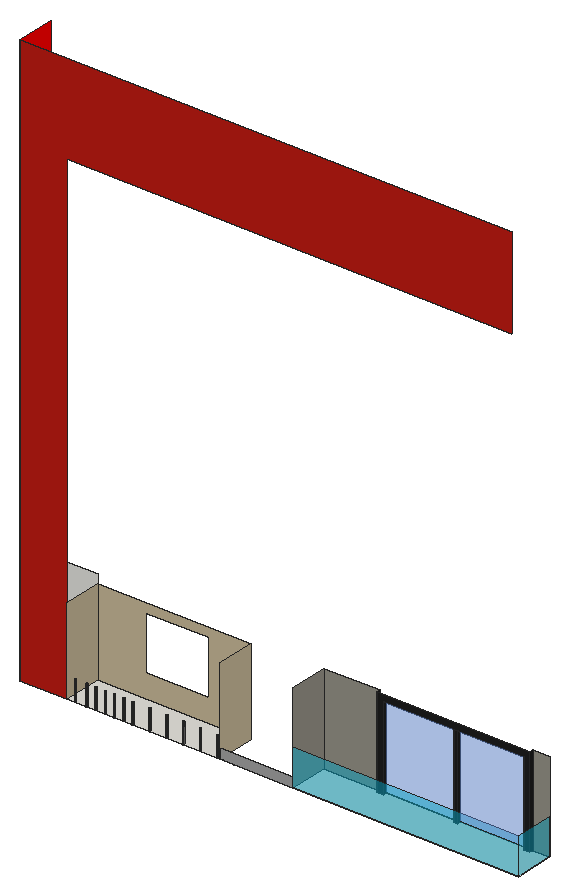
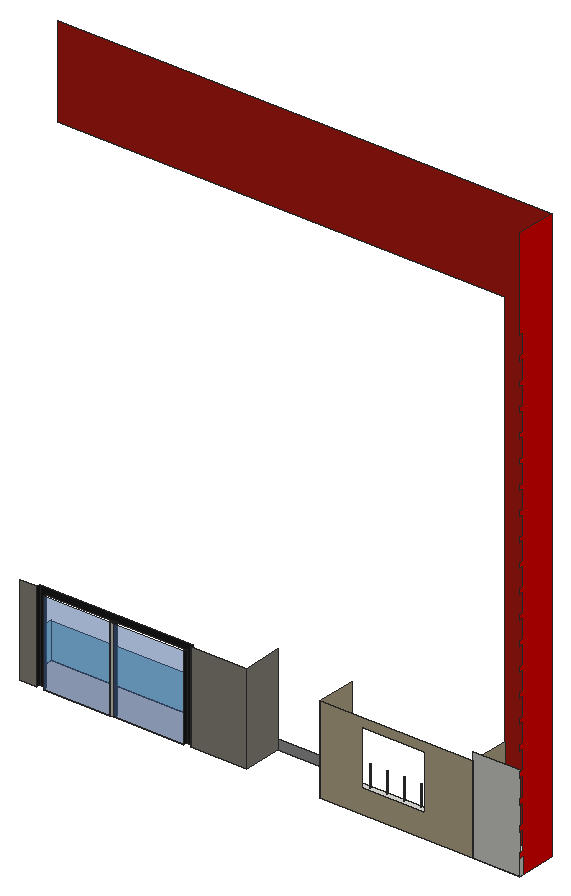
# SketchUp Ruby script. Lengths in inches.
U = 1.inch
M = Sketchup.active_model
def pt(a) = Geom::Point3d.new(a.map { |v| v * U })
def face(e, loops, mat)
  f = e.add_face(loops[0].map { |a| pt(a) })
  loops[1..].each { |l| e.add_face(l.map { |a| pt(a) }).erase! }
  f.material = f.back_material = mat if mat
  f
end
# faces: each face lists its corners as indices into pts; further lists are holes
def faces(e, pts, list, mat = nil) = list.each { |f| face(e, (f[0].is_a?(Array) ? f : [f]).map { |l| l.map { |i| pts[i] } }, mat) }
# xy, xz, yz: faces in a plane at the given z, y or x. An outline is a flat list of corners, or four numbers for a rectangle; further outlines are holes
def ring(l) = l.size == 4 ? [[l[0], l[1]], [l[2], l[1]], [l[2], l[3]], [l[0], l[3]]] : l.each_slice(2).to_a
def flat(e, list, mat, &to3) = list.each { |f| face(e, (f[0].is_a?(Array) ? f : [f]).map { |l| ring(l).map { |u, v| to3.(u, v) } }, mat) }
def xy(e, z, list, mat = nil) = flat(e, list, mat) { |x, y| [x, y, z] }
def xz(e, y, list, mat = nil) = flat(e, list, mat) { |x, z| [x, y, z] }
def yz(e, x, list, mat = nil) = flat(e, list, mat) { |y, z| [x, y, z] }
def lines(e, pts, list) = list.each { |a, b| e.add_line(pt(pts[a]), pt(pts[b])) }
# prism: a flat outline (further loops are holes) pulled along v
def prism(e, loops, v, mat = nil)
  f = face(e, loops, mat); d = Geom::Vector3d.new(v.map { |x| x * U })
  f.pushpull(f.normal.samedirection?(d) ? d.length : -d.length)
end
def box(e, o, s, mat = nil) = prism(e, [[o, [o[0] + s[0], o[1], o[2]], [o[0] + s[0], o[1] + s[1], o[2]], [o[0], o[1] + s[1], o[2]]]], [0, 0, s[2]], mat)
def at(x, y, z, deg = 0) = Geom::Transformation.translation(pt([x, y, z])) * Geom::Transformation.rotation(ORIGIN, Z_AXIS, deg.degrees)
def axes(o, x, y, z) = Geom::Transformation.new([*x, 0, *y, 0, *z, 0, *pt(o).to_a, 1])
def part(name) = M.definitions.add(name)
# library, detail: a bought-in or finely detailed component or shape, given as its bounding box
def library(name, o, s) = part(name).tap { |d| box(d.entities, o, s) }
def detail(e, o, s) = box(e.add_group.entities, o, s)
def put(e, d, t, mat = nil) = e.add_instance(d, t).tap { |i| i.material = mat if mat }
def group(e, t, mat = nil) = e.add_group.tap { |g| g.transformation = t; g.material = mat if mat }.entities
root = M.entities
M.materials.add("[0020_Red]").color = [255, 0, 0]
M.materials.add("[0133_Gray]").color = [128, 128, 128]
M.materials.add("[Blacktop New]").color = [30, 30, 30]
M.materials.add("[Formica Graystone]").color = [149, 146, 135]
M.materials.add("[Marble Carrara Gold Floor Tile]").color = [225, 223, 217]
M.materials.add("[Modern Siding]").color = [191, 28, 19]
M.materials.add("[Pavers Flagstone Gray]").color = [162, 162, 162]
M.materials.add("[Quartz Light Brown]").color = [199, 184, 152]
M.materials.add("[Translucent Glass Blue]").color = [100, 149, 237]
M.materials["[Translucent Glass Blue]"].alpha = 0.5
M.materials.add("[Translucent Glass Tinted]").color = [8, 201, 241]
M.materials["[Translucent Glass Tinted]"].alpha = 0.48
xy(root,151.96,[[45.0625,3,88.53,39],[242.69,3.4,242.82,3.4,242.94,3.44,243.05,3.52,243.14,3.61,243.2,3.73,243.22,3.86,243.22,3.99,243.18,4.11,243.1,4.22,243.01,4.31,242.89,4.37,242.76,4.39,242.63,4.39,242.51,4.34,242.4,4.27,242.3125,4.18,242.25,4.06,242.23,3.93,242.23,3.8,242.28,3.68,242.35,3.57,242.45,3.48,242.5625,3.42],[420.16,36,423.8,39]])
xy(root,151.96,[[[88.53,3,229.62,39],[95.31,3.4,95.1875,3.42,95.07,3.48,94.97,3.57,94.9,3.68,94.86,3.8,94.85,3.93,94.88,4.06,94.9375,4.18,95.02,4.27,95.13,4.34,95.26,4.39,95.39,4.39,95.51,4.37,95.63,4.31,95.73,4.22,95.8,4.11,95.84,3.99,95.85,3.86,95.82,3.73,95.76,3.61,95.68,3.52,95.57,3.44,95.45,3.4],[106.13,3.4,106,3.42,105.88,3.48,105.79,3.57,105.71,3.68,105.67,3.8,105.66,3.93,105.69,4.06,105.75,4.18,105.84,4.27,105.94,4.34,106.07,4.39,106.2,4.39,106.33,4.37,106.44,4.31,106.54,4.22,106.61,4.11,106.65,3.99,106.66,3.86,106.64,3.73,106.58,3.61,106.49,3.52,106.38,3.44,106.26,3.4],[114.69,3.4,114.5625,3.42,114.45,3.48,114.35,3.57,114.28,3.68,114.23,3.8,114.23,3.93,114.25,4.06,114.3125,4.18,114.4,4.27,114.51,4.34,114.63,4.39,114.76,4.39,114.89,4.37,115.01,4.31,115.1,4.22,115.18,4.11,115.22,3.99,115.22,3.86,115.2,3.73,115.14,3.61,115.05,3.52,114.94,3.44,114.82,3.4],[123.25,3.4,123.125,3.42,123.01,3.48,122.91,3.57,122.84,3.68,122.8,3.8,122.79,3.93,122.82,4.06,122.875,4.18,122.96,4.27,123.07,4.34,123.19,4.39,123.32,4.39,123.45,4.37,123.57,4.31,123.67,4.22,123.74,4.11,123.78,3.99,123.79,3.86,123.76,3.73,123.7,3.61,123.62,3.52,123.51,3.44,123.38,3.4],[131.81,3.4,131.6875,3.42,131.57,3.48,131.47,3.57,131.4,3.68,131.36,3.8,131.35,3.93,131.38,4.06,131.4375,4.18,131.52,4.27,131.63,4.34,131.76,4.39,131.89,4.39,132.01,4.37,132.13,4.31,132.23,4.22,132.3,4.11,132.34,3.99,132.35,3.86,132.32,3.73,132.26,3.61,132.18,3.52,132.07,3.44,131.95,3.4],[140.38,3.4,140.25,3.42,140.13,3.48,140.04,3.57,139.96,3.68,139.92,3.8,139.91,3.93,139.94,4.06,140,4.18,140.09,4.27,140.19,4.34,140.32,4.39,140.45,4.39,140.58,4.37,140.69,4.31,140.79,4.22,140.86,4.11,140.9,3.99,140.91,3.86,140.89,3.73,140.83,3.61,140.74,3.52,140.63,3.44,140.51,3.4],[148.94,3.4,148.8125,3.42,148.7,3.48,148.6,3.57,148.53,3.68,148.48,3.8,148.48,3.93,148.5,4.06,148.5625,4.18,148.65,4.27,148.76,4.34,148.88,4.39,149.01,4.39,149.14,4.37,149.26,4.31,149.35,4.22,149.43,4.11,149.47,3.99,149.47,3.86,149.45,3.73,149.39,3.61,149.3,3.52,149.19,3.44,149.07,3.4],[164.56,3.4,164.4375,3.42,164.32,3.48,164.22,3.57,164.15,3.68,164.11,3.8,164.1,3.93,164.13,4.06,164.1875,4.18,164.27,4.27,164.38,4.34,164.51,4.39,164.64,4.39,164.76,4.37,164.88,4.31,164.98,4.22,165.05,4.11,165.09,3.99,165.1,3.86,165.07,3.73,165.01,3.61,164.93,3.52,164.82,3.44,164.7,3.4],[180.19,3.4,180.0625,3.42,179.95,3.48,179.85,3.57,179.78,3.68,179.73,3.8,179.73,3.93,179.75,4.06,179.8125,4.18,179.9,4.27,180.01,4.34,180.13,4.39,180.26,4.39,180.39,4.37,180.51,4.31,180.6,4.22,180.68,4.11,180.72,3.99,180.72,3.86,180.7,3.73,180.64,3.61,180.55,3.52,180.44,3.44,180.32,3.4],[195.81,3.4,195.6875,3.42,195.57,3.48,195.47,3.57,195.4,3.68,195.36,3.8,195.35,3.93,195.38,4.06,195.4375,4.18,195.52,4.27,195.63,4.34,195.76,4.39,195.89,4.39,196.01,4.37,196.13,4.31,196.23,4.22,196.3,4.11,196.34,3.99,196.35,3.86,196.32,3.73,196.26,3.61,196.18,3.52,196.07,3.44,195.95,3.4],[211.44,3.4,211.3125,3.42,211.2,3.48,211.1,3.57,211.03,3.68,210.98,3.8,210.98,3.93,211,4.06,211.0625,4.18,211.15,4.27,211.26,4.34,211.38,4.39,211.51,4.39,211.64,4.37,211.76,4.31,211.85,4.22,211.93,4.11,211.97,3.99,211.97,3.86,211.95,3.73,211.89,3.61,211.8,3.52,211.69,3.44,211.57,3.4],[227.06,3.4,226.9375,3.42,226.82,3.48,226.72,3.57,226.65,3.68,226.61,3.8,226.6,3.93,226.63,4.06,226.6875,4.18,226.77,4.27,226.88,4.34,227.01,4.39,227.14,4.39,227.26,4.37,227.38,4.31,227.48,4.22,227.55,4.11,227.59,3.99,227.6,3.86,227.57,3.73,227.51,3.61,227.43,3.52,227.32,3.44,227.2,3.4]],[297.58,3,506.625,3,506.625,39,491,39,491,36,485,36,485,39,423.8,39,423.8,36,420.16,36,420.16,39,355.33,39,355.33,36,349.33,36,349.33,39,297.58,39]],"[Marble Carrara Gold Floor Tile]")
xz(root,3,[[45.0625,151.96,88.53,151.96,88.53,600,500.56,600,500.56,683.96,45.0625,683.96]],"[Modern Siding]")
xz(root,3,[[229.62,151.96,297.58,161.3125]],"[Pavers Flagstone Gray]")
xz(root,3,[[297.58,151.96,506.625,185.64]],"[Translucent Glass Tinted]")
xz(root,3.4,[[95.31,151.96,95.45,170.4],[106.13,151.96,106.26,170.77],[114.69,151.96,114.82,170.77],[123.25,151.96,123.38,170.77],[131.81,151.96,131.95,170.77],
  [140.38,151.96,140.51,170.77],[148.94,151.96,149.07,170.77],[164.56,151.96,164.7,170.77],[180.19,151.96,180.32,170.77],[195.81,151.96,195.95,170.77],
  [211.44,151.96,211.57,170.77],[227.06,151.96,227.2,170.77]],"[0133_Gray]")
xz(root,4.39,[[95.26,151.96,95.39,170.4],[106.07,151.96,106.2,170.77],[114.63,151.96,114.76,170.77],[123.19,151.96,123.32,170.77],[131.76,151.96,131.89,170.77],
  [140.32,151.96,140.45,170.77],[148.88,151.96,149.01,170.77],[164.51,151.96,164.64,170.77],[180.13,151.96,180.26,170.77],[195.76,151.96,195.89,170.77],
  [211.38,151.96,211.51,170.77],[227.01,151.96,227.14,170.77]],"[0133_Gray]")
xz(root,36,[[349.33,151.96,355.33,151.96,355.33,229.1875,485,229.1875,485,151.96,491,151.96,491,235.1875,349.33,235.1875],[420.16,151.96,423.8,229.1875]],"[Blacktop New]")
xz(root,39,[[45.0625,151.96,88.53,240],[420.16,151.96,423.8,229.1875]])
xz(root,39,[[297.58,151.96,349.33,235.1875],[491,151.96,506.625,235.1875]],"[Formica Graystone]")
xz(root,39,[[[88.53,151.96,229.62,232],[133.06,173.78,191.5,223.84]]],"[Quartz Light Brown]")
xz(root,39,[[355.33,151.96,420.16,229.1875],[423.8,151.96,485,229.1875]],"[Translucent Glass Blue]")
yz(root,45.0625,[[36,151.96,39,166.5625]])
yz(root,45.0625,[[3,151.96,3,683.96,39,683.96,39,600,36,600,36,582.64,39,582.64,39,578.5625,36,578.5625,36,561.2,39,561.2,39,557.125,36,557.125,36,539.76,39,539.76,39,535.6875,36,535.6875,36,518.32,39,518.32,39,514.25,36,514.25,36,496.89,39,496.89,39,492.8125,36,492.8125,36,475.45,39,475.45,39,471.375,36,471.375,36,454.01,39,454.01,39,449.9375,36,449.9375,36,432.57,39,432.57,39,428.5,36,428.5,36,411.14,39,411.14,39,407.0625,36,407.0625,36,389.7,39,389.7,39,385.625,36,385.625,36,368.26,39,368.26,39,364.1875,36,364.1875,36,346.82,39,346.82,39,342.75,36,342.75,36,325.39,39,325.39,39,321.3125,36,321.3125,36,303.95,39,303.95,39,299.875,36,299.875,36,282.51,39,282.51,39,278.4375,36,278.4375,36,261.07,39,261.07,39,256.0625,36,256.0625,36,238.7,39,238.7,39,233.6875,36,233.6875,36,216.32,39,216.32,39,211.3125,36,211.3125,36,193.95,39,193.95,39,188.9375,36,188.9375,36,171.57,39,171.57,39,166.5625,36,166.5625,36,151.96]],"[0020_Red]")
yz(root,88.53,[[[3,151.96,39,232],[4.01,154.41,3.84,154.43,3.69,154.49,3.5625,154.59,3.46,154.72,3.4,154.87,3.38,155.03,3.4,155.19,3.46,155.34,3.5625,155.47,3.69,155.57,3.84,155.64,4.01,155.66,4.17,155.64,4.32,155.57,4.45,155.47,4.55,155.34,4.61,155.19,4.63,155.03,4.61,154.87,4.55,154.72,4.45,154.59,4.32,154.49,4.17,154.43],[4.01,156.41,3.84,156.43,3.69,156.49,3.5625,156.59,3.46,156.72,3.4,156.87,3.38,157.03,3.4,157.19,3.46,157.34,3.5625,157.47,3.69,157.57,3.84,157.64,4.01,157.66,4.17,157.64,4.32,157.57,4.45,157.47,4.55,157.34,4.61,157.19,4.63,157.03,4.61,156.87,4.55,156.72,4.45,156.59,4.32,156.49,4.17,156.43],[4.01,158.41,3.84,158.43,3.69,158.49,3.5625,158.59,3.46,158.72,3.4,158.87,3.38,159.03,3.4,159.19,3.46,159.34,3.5625,159.47,3.69,159.57,3.84,159.64,4.01,159.66,4.17,159.64,4.32,159.57,4.45,159.47,4.55,159.34,4.61,159.19,4.63,159.03,4.61,158.87,4.55,158.72,4.45,158.59,4.32,158.49,4.17,158.43],[4.01,160.41,3.84,160.43,3.69,160.49,3.5625,160.59,3.46,160.72,3.4,160.87,3.38,161.03,3.4,161.19,3.46,161.34,3.5625,161.47,3.69,161.57,3.84,161.64,4.01,161.66,4.17,161.64,4.32,161.57,4.45,161.47,4.55,161.34,4.61,161.19,4.63,161.03,4.61,160.87,4.55,160.72,4.45,160.59,4.32,160.49,4.17,160.43],[4.01,162.41,3.84,162.43,3.69,162.49,3.5625,162.59,3.46,162.72,3.4,162.87,3.38,163.03,3.4,163.19,3.46,163.34,3.5625,163.47,3.69,163.57,3.84,163.64,4.01,163.66,4.17,163.64,4.32,163.57,4.45,163.47,4.55,163.34,4.61,163.19,4.63,163.03,4.61,162.87,4.55,162.72,4.45,162.59,4.32,162.49,4.17,162.43],[4.01,164.41,3.84,164.43,3.69,164.49,3.5625,164.59,3.46,164.72,3.4,164.87,3.38,165.03,3.4,165.19,3.46,165.34,3.5625,165.47,3.69,165.57,3.84,165.64,4.01,165.66,4.17,165.64,4.32,165.57,4.45,165.47,4.55,165.34,4.61,165.19,4.63,165.03,4.61,164.87,4.55,164.72,4.45,164.59,4.32,164.49,4.17,164.43],[4.01,166.41,3.84,166.43,3.69,166.49,3.5625,166.59,3.46,166.72,3.4,166.87,3.38,167.03,3.4,167.19,3.46,167.34,3.5625,167.47,3.69,167.57,3.84,167.64,4.01,167.66,4.17,167.64,4.32,167.57,4.45,167.47,4.55,167.34,4.61,167.19,4.63,167.03,4.61,166.87,4.55,166.72,4.45,166.59,4.32,166.49,4.17,166.43],[4.01,168.41,3.84,168.43,3.69,168.49,3.5625,168.59,3.46,168.72,3.4,168.87,3.38,169.03,3.4,169.19,3.46,169.34,3.5625,169.47,3.69,169.57,3.84,169.64,4.01,169.66,4.17,169.64,4.32,169.57,4.45,169.47,4.55,169.34,4.61,169.19,4.63,169.03,4.61,168.87,4.55,168.72,4.45,168.59,4.32,168.49,4.17,168.43]]],"[Quartz Light Brown]")
yz(root,114.23,[[3.8,151.96,3.93,170.77]],"[0133_Gray]")
yz(root,115.22,[[3.86,151.96,3.99,170.77]],"[0133_Gray]")
yz(root,148.48,[[3.8,151.96,3.93,170.77]],"[0133_Gray]")
yz(root,149.47,[[3.86,151.96,3.99,170.77]],"[0133_Gray]")
yz(root,179.73,[[3.8,151.96,3.93,170.77]],"[0133_Gray]")
yz(root,180.72,[[3.86,151.96,3.99,170.77]],"[0133_Gray]")
yz(root,210.98,[[3.8,151.96,3.93,170.77]],"[0133_Gray]")
yz(root,211.97,[[3.86,151.96,3.99,170.77]],"[0133_Gray]")
yz(root,229.62,[[[3,151.96,39,232],[4.01,160.41,4.17,160.43,4.32,160.49,4.45,160.59,4.55,160.72,4.61,160.87,4.63,161.03,4.61,161.19,4.55,161.34,4.45,161.47,4.32,161.57,4.17,161.64,4.01,161.66,3.84,161.64,3.69,161.57,3.5625,161.47,3.46,161.34,3.4,161.19,3.38,161.03,3.4,160.87,3.46,160.72,3.5625,160.59,3.69,160.49,3.84,160.43]]],"[Quartz Light Brown]")
yz(root,232.85,[[4.01,152.41,4.17,152.43,4.32,152.49,4.45,152.59,4.55,152.72,4.61,152.87,4.63,153.03,4.61,153.19,4.55,153.34,4.45,153.47,4.32,153.57,4.17,153.64,4.01,153.66,3.84,153.64,3.69,153.57,3.5625,153.47,3.46,153.34,3.4,153.19,3.38,153.03,3.4,152.87,3.46,152.72,3.5625,152.59,3.69,152.49,3.84,152.43]])
yz(root,297.58,[[3,151.96,39,235.1875]],"[Formica Graystone]")
yz(root,349.33,[[36,151.96,39,235.1875]],"[Blacktop New]")
yz(root,355.33,[[36,151.96,39,229.1875]],"[Blacktop New]")
yz(root,420.16,[[36,151.96,39,229.1875]],"[Blacktop New]")
yz(root,423.8,[[36,151.96,39,229.1875]],"[Blacktop New]")
yz(root,485,[[36,151.96,39,229.1875]],"[Blacktop New]")
yz(root,491,[[36,151.96,39,235.1875]],"[Blacktop New]")
yz(root,506.625,[[3,151.96,39,185.75]],"[Translucent Glass Tinted]")
p = [[95.07,3.48,151.96],[95.1875,3.42,151.96],[95.1875,3.42,170.4],[95.07,3.48,170.4],[95.31,3.4,151.96],[95.31,3.4,170.4],
  [95.45,3.4,151.96],[95.57,3.44,151.96],[95.57,3.44,170.4],[95.45,3.4,170.4],[95.68,3.52,151.96],[95.68,3.52,170.4],
  [105.88,3.48,151.96],[106,3.42,151.96],[106,3.42,170.77],[105.88,3.48,170.77],[106.13,3.4,151.96],[106.13,3.4,170.77],
  [106.26,3.4,151.96],[106.38,3.44,151.96],[106.38,3.44,170.77],[106.26,3.4,170.77],[106.49,3.52,151.96],[106.49,3.52,170.77],
  [114.45,3.48,151.96],[114.5625,3.42,151.96],[114.5625,3.42,170.77],[114.45,3.48,170.77],[114.69,3.4,151.96],[114.69,3.4,170.77],
  [114.82,3.4,151.96],[114.94,3.44,151.96],[114.94,3.44,170.77],[114.82,3.4,170.77],[115.05,3.52,151.96],[115.05,3.52,170.77],
  [123.01,3.48,151.96],[123.125,3.42,151.96],[123.125,3.42,170.77],[123.01,3.48,170.77],[123.25,3.4,151.96],[123.25,3.4,170.77],
  [123.38,3.4,151.96],[123.51,3.44,151.96],[123.51,3.44,170.77],[123.38,3.4,170.77],[123.62,3.52,151.96],[123.62,3.52,170.77],
  [131.57,3.48,151.96],[131.6875,3.42,151.96],[131.6875,3.42,170.77],[131.57,3.48,170.77],[131.81,3.4,151.96],[131.81,3.4,170.77],
  [131.95,3.4,151.96],[132.07,3.44,151.96],[132.07,3.44,170.77],[131.95,3.4,170.77],[132.18,3.52,151.96],[132.18,3.52,170.77],
  [140.13,3.48,151.96],[140.25,3.42,151.96],[140.25,3.42,170.77],[140.13,3.48,170.77],[140.38,3.4,151.96],[140.38,3.4,170.77],
  [140.51,3.4,151.96],[140.63,3.44,151.96],[140.63,3.44,170.77],[140.51,3.4,170.77],[140.74,3.52,151.96],[140.74,3.52,170.77],
  [148.7,3.48,151.96],[148.8125,3.42,151.96],[148.8125,3.42,170.77],[148.7,3.48,170.77],[148.94,3.4,151.96],[148.94,3.4,170.77],
  [149.07,3.4,151.96],[149.19,3.44,151.96],[149.19,3.44,170.77],[149.07,3.4,170.77],[149.3,3.52,151.96],[149.3,3.52,170.77],
  [164.32,3.48,151.96],[164.4375,3.42,151.96],[164.4375,3.42,170.77],[164.32,3.48,170.77],[164.56,3.4,151.96],[164.56,3.4,170.77],
  [164.7,3.4,151.96],[164.82,3.44,151.96],[164.82,3.44,170.77],[164.7,3.4,170.77],[164.93,3.52,151.96],[164.93,3.52,170.77],
  [179.95,3.48,151.96],[180.0625,3.42,151.96],[180.0625,3.42,170.77],[179.95,3.48,170.77],[180.19,3.4,151.96],[180.19,3.4,170.77],
  [180.32,3.4,151.96],[180.44,3.44,151.96],[180.44,3.44,170.77],[180.32,3.4,170.77],[180.55,3.52,151.96],[180.55,3.52,170.77],
  [195.57,3.48,151.96],[195.6875,3.42,151.96],[195.6875,3.42,170.77],[195.57,3.48,170.77],[195.81,3.4,151.96],[195.81,3.4,170.77],
  [195.95,3.4,151.96],[196.07,3.44,151.96],[196.07,3.44,170.77],[195.95,3.4,170.77],[196.18,3.52,151.96],[196.18,3.52,170.77],
  [211.2,3.48,151.96],[211.3125,3.42,151.96],[211.3125,3.42,170.77],[211.2,3.48,170.77],[211.44,3.4,151.96],[211.44,3.4,170.77],
  [211.57,3.4,151.96],[211.69,3.44,151.96],[211.69,3.44,170.77],[211.57,3.4,170.77],[211.8,3.52,151.96],[211.8,3.52,170.77],
  [226.82,3.48,151.96],[226.9375,3.42,151.96],[226.9375,3.42,170.77],[226.82,3.48,170.77],[227.06,3.4,151.96],[227.06,3.4,170.77],
  [227.2,3.4,151.96],[227.32,3.44,151.96],[227.32,3.44,170.77],[227.2,3.4,170.77],[227.43,3.52,151.96],[227.43,3.52,170.77],
  [94.97,3.57,151.96],[94.97,3.57,170.4],[95.76,3.61,151.96],[95.76,3.61,170.4],[105.79,3.57,151.96],[105.79,3.57,170.77],
  [106.58,3.61,151.96],[106.58,3.61,170.77],[114.35,3.57,151.96],[114.35,3.57,170.77],[115.14,3.61,151.96],[115.14,3.61,170.77],
  [122.91,3.57,151.96],[122.91,3.57,170.77],[123.7,3.61,151.96],[123.7,3.61,170.77],[131.47,3.57,151.96],[131.47,3.57,170.77],
  [132.26,3.61,151.96],[132.26,3.61,170.77],[140.04,3.57,151.96],[140.04,3.57,170.77],[140.83,3.61,151.96],[140.83,3.61,170.77],
  [148.6,3.57,151.96],[148.6,3.57,170.77],[149.39,3.61,151.96],[149.39,3.61,170.77],[164.22,3.57,151.96],[164.22,3.57,170.77],
  [165.01,3.61,151.96],[165.01,3.61,170.77],[179.85,3.57,151.96],[179.85,3.57,170.77],[180.64,3.61,151.96],[180.64,3.61,170.77],
  [195.47,3.57,151.96],[195.47,3.57,170.77],[196.26,3.61,151.96],[196.26,3.61,170.77],[211.1,3.57,151.96],[211.1,3.57,170.77],
  [211.89,3.61,151.96],[211.89,3.61,170.77],[226.72,3.57,151.96],[226.72,3.57,170.77],[227.51,3.61,151.96],[227.51,3.61,170.77],
  [94.9,3.68,151.96],[94.9,3.68,170.4],[95.82,3.73,151.96],[95.82,3.73,170.4],[105.71,3.68,151.96],[105.71,3.68,170.77],
  [106.64,3.73,151.96],[106.64,3.73,170.77],[114.28,3.68,151.96],[114.28,3.68,170.77],[115.2,3.73,151.96],[115.2,3.73,170.77],
  [122.84,3.68,151.96],[122.84,3.68,170.77],[123.76,3.73,151.96],[123.76,3.73,170.77],[131.4,3.68,151.96],[131.4,3.68,170.77],
  [132.32,3.73,151.96],[132.32,3.73,170.77],[139.96,3.68,151.96],[139.96,3.68,170.77],[140.89,3.73,151.96],[140.89,3.73,170.77],
  [148.53,3.68,151.96],[148.53,3.68,170.77],[149.45,3.73,151.96],[149.45,3.73,170.77],[164.15,3.68,151.96],[164.15,3.68,170.77],
  [165.07,3.73,151.96],[165.07,3.73,170.77],[179.78,3.68,151.96],[179.78,3.68,170.77],[180.7,3.73,151.96],[180.7,3.73,170.77],
  [195.4,3.68,151.96],[195.4,3.68,170.77],[196.32,3.73,151.96],[196.32,3.73,170.77],[211.03,3.68,151.96],[211.03,3.68,170.77],
  [211.95,3.73,151.96],[211.95,3.73,170.77],[226.65,3.68,151.96],[226.65,3.68,170.77],[227.57,3.73,151.96],[227.57,3.73,170.77],
  [94.86,3.8,151.96],[94.86,3.8,170.4],[95.85,3.86,151.96],[95.85,3.86,170.4],[105.67,3.8,151.96],[105.67,3.8,170.77],
  [106.66,3.86,151.96],[106.66,3.86,170.77],[114.23,3.8,151.96],[114.23,3.8,170.77],[115.22,3.86,151.96],[115.22,3.86,170.77],
  [122.8,3.8,151.96],[122.8,3.8,170.77],[123.79,3.86,151.96],[123.79,3.86,170.77],[131.36,3.8,151.96],[131.36,3.8,170.77],
  [132.35,3.86,151.96],[132.35,3.86,170.77],[139.92,3.8,151.96],[139.92,3.8,170.77],[140.91,3.86,151.96],[140.91,3.86,170.77],
  [148.48,3.8,151.96],[148.48,3.8,170.77],[149.47,3.86,151.96],[149.47,3.86,170.77],[164.11,3.8,151.96],[164.11,3.8,170.77],
  [165.1,3.86,151.96],[165.1,3.86,170.77],[179.73,3.8,151.96],[179.73,3.8,170.77],[180.72,3.86,151.96],[180.72,3.86,170.77],
  [195.36,3.8,151.96],[195.36,3.8,170.77],[196.35,3.86,151.96],[196.35,3.86,170.77],[210.98,3.8,151.96],[210.98,3.8,170.77],
  [211.97,3.86,151.96],[211.97,3.86,170.77],[226.61,3.8,151.96],[226.61,3.8,170.77],[227.6,3.86,151.96],[227.6,3.86,170.77],
  [94.85,3.93,151.96],[94.85,3.93,170.4],[105.66,3.93,151.96],[105.66,3.93,170.77],[122.79,3.93,151.96],[122.79,3.93,170.77],
  [131.35,3.93,151.96],[131.35,3.93,170.77],[139.91,3.93,151.96],[139.91,3.93,170.77],[164.1,3.93,151.96],[164.1,3.93,170.77],
  [195.35,3.93,151.96],[195.35,3.93,170.77],[226.6,3.93,151.96],[226.6,3.93,170.77],[94.88,4.06,151.96],[94.88,4.06,170.4],
  [95.84,3.99,151.96],[95.84,3.99,170.4],[105.69,4.06,151.96],[105.69,4.06,170.77],[106.65,3.99,151.96],[106.65,3.99,170.77],
  [114.25,4.06,151.96],[114.23,3.93,151.96],[114.23,3.93,170.77],[114.25,4.06,170.77],[122.82,4.06,151.96],[122.82,4.06,170.77],
  [123.78,3.99,151.96],[123.78,3.99,170.77],[131.38,4.06,151.96],[131.38,4.06,170.77],[132.34,3.99,151.96],[132.34,3.99,170.77],
  [139.94,4.06,151.96],[139.94,4.06,170.77],[140.9,3.99,151.96],[140.9,3.99,170.77],[148.5,4.06,151.96],[148.48,3.93,151.96],
  [148.48,3.93,170.77],[148.5,4.06,170.77],[164.13,4.06,151.96],[164.13,4.06,170.77],[165.09,3.99,151.96],[165.09,3.99,170.77],
  [179.75,4.06,151.96],[179.73,3.93,151.96],[179.73,3.93,170.77],[179.75,4.06,170.77],[195.38,4.06,151.96],[195.38,4.06,170.77],
  [196.34,3.99,151.96],[196.34,3.99,170.77],[211,4.06,151.96],[210.98,3.93,151.96],[210.98,3.93,170.77],[211,4.06,170.77],
  [226.63,4.06,151.96],[226.63,4.06,170.77],[227.59,3.99,151.96],[227.59,3.99,170.77],[95.8,4.11,151.96],[95.8,4.11,170.4],
  [106.61,4.11,151.96],[106.61,4.11,170.77],[115.22,3.99,151.96],[115.18,4.11,151.96],[115.18,4.11,170.77],[115.22,3.99,170.77],
  [123.74,4.11,151.96],[123.74,4.11,170.77],[132.3,4.11,151.96],[132.3,4.11,170.77],[140.86,4.11,151.96],[140.86,4.11,170.77],
  [149.47,3.99,151.96],[149.43,4.11,151.96],[149.43,4.11,170.77],[149.47,3.99,170.77],[165.05,4.11,151.96],[165.05,4.11,170.77],
  [180.72,3.99,151.96],[180.68,4.11,151.96],[180.68,4.11,170.77],[180.72,3.99,170.77],[196.3,4.11,151.96],[196.3,4.11,170.77],
  [211.97,3.99,151.96],[211.93,4.11,151.96],[211.93,4.11,170.77],[211.97,3.99,170.77],[227.55,4.11,151.96],[227.55,4.11,170.77],
  [94.9375,4.18,151.96],[94.9375,4.18,170.4],[95.73,4.22,151.96],[95.73,4.22,170.4],[105.75,4.18,151.96],[105.75,4.18,170.77],
  [106.54,4.22,151.96],[106.54,4.22,170.77],[114.3125,4.18,151.96],[114.3125,4.18,170.77],[115.1,4.22,151.96],[115.1,4.22,170.77],
  [122.875,4.18,151.96],[122.875,4.18,170.77],[123.67,4.22,151.96],[123.67,4.22,170.77],[131.4375,4.18,151.96],[131.4375,4.18,170.77],
  [132.23,4.22,151.96],[132.23,4.22,170.77],[140,4.18,151.96],[140,4.18,170.77],[140.79,4.22,151.96],[140.79,4.22,170.77],
  [148.5625,4.18,151.96],[148.5625,4.18,170.77],[149.35,4.22,151.96],[149.35,4.22,170.77],[164.1875,4.18,151.96],[164.1875,4.18,170.77],
  [164.98,4.22,151.96],[164.98,4.22,170.77],[179.8125,4.18,151.96],[179.8125,4.18,170.77],[180.6,4.22,151.96],[180.6,4.22,170.77],
  [195.4375,4.18,151.96],[195.4375,4.18,170.77],[196.23,4.22,151.96],[196.23,4.22,170.77],[211.0625,4.18,151.96],[211.0625,4.18,170.77],
  [211.85,4.22,151.96],[211.85,4.22,170.77],[226.6875,4.18,151.96],[226.6875,4.18,170.77],[227.48,4.22,151.96],[227.48,4.22,170.77],
  [95.02,4.27,151.96],[95.02,4.27,170.4],[95.63,4.31,151.96],[95.63,4.31,170.4],[105.84,4.27,151.96],[105.84,4.27,170.77],
  [106.44,4.31,151.96],[106.44,4.31,170.77],[114.4,4.27,151.96],[114.4,4.27,170.77],[115.01,4.31,151.96],[115.01,4.31,170.77],
  [122.96,4.27,151.96],[122.96,4.27,170.77],[123.57,4.31,151.96],[123.57,4.31,170.77],[131.52,4.27,151.96],[131.52,4.27,170.77],
  [132.13,4.31,151.96],[132.13,4.31,170.77],[140.09,4.27,151.96],[140.09,4.27,170.77],[140.69,4.31,151.96],[140.69,4.31,170.77],
  [148.65,4.27,151.96],[148.65,4.27,170.77],[149.26,4.31,151.96],[149.26,4.31,170.77],[164.27,4.27,151.96],[164.27,4.27,170.77],
  [164.88,4.31,151.96],[164.88,4.31,170.77],[179.9,4.27,151.96],[179.9,4.27,170.77],[180.51,4.31,151.96],[180.51,4.31,170.77],
  [195.52,4.27,151.96],[195.52,4.27,170.77],[196.13,4.31,151.96],[196.13,4.31,170.77],[211.15,4.27,151.96],[211.15,4.27,170.77],
  [211.76,4.31,151.96],[211.76,4.31,170.77],[226.77,4.27,151.96],[226.77,4.27,170.77],[227.38,4.31,151.96],[227.38,4.31,170.77],
  [95.13,4.34,151.96],[95.13,4.34,170.4],[95.26,4.39,151.96],[95.26,4.39,170.4],[95.51,4.37,151.96],[95.51,4.37,170.4],
  [105.94,4.34,151.96],[105.94,4.34,170.77],[106.07,4.39,151.96],[106.07,4.39,170.77],[106.33,4.37,151.96],[106.33,4.37,170.77],
  [114.51,4.34,151.96],[114.51,4.34,170.77],[114.63,4.39,151.96],[114.63,4.39,170.77],[114.89,4.37,151.96],[114.89,4.37,170.77],
  [123.07,4.34,151.96],[123.07,4.34,170.77],[123.19,4.39,151.96],[123.19,4.39,170.77],[123.45,4.37,151.96],[123.45,4.37,170.77],
  [131.63,4.34,151.96],[131.63,4.34,170.77],[131.76,4.39,151.96],[131.76,4.39,170.77],[132.01,4.37,151.96],[132.01,4.37,170.77],
  [140.19,4.34,151.96],[140.19,4.34,170.77],[140.32,4.39,151.96],[140.32,4.39,170.77],[140.58,4.37,151.96],[140.58,4.37,170.77],
  [148.76,4.34,151.96],[148.76,4.34,170.77],[148.88,4.39,151.96],[148.88,4.39,170.77],[149.14,4.37,151.96],[149.14,4.37,170.77],
  [164.38,4.34,151.96],[164.38,4.34,170.77],[164.51,4.39,151.96],[164.51,4.39,170.77],[164.76,4.37,151.96],[164.76,4.37,170.77],
  [180.01,4.34,151.96],[180.01,4.34,170.77],[180.13,4.39,151.96],[180.13,4.39,170.77],[180.39,4.37,151.96],[180.39,4.37,170.77],
  [195.63,4.34,151.96],[195.63,4.34,170.77],[195.76,4.39,151.96],[195.76,4.39,170.77],[196.01,4.37,151.96],[196.01,4.37,170.77],
  [211.26,4.34,151.96],[211.26,4.34,170.77],[211.38,4.39,151.96],[211.38,4.39,170.77],[211.64,4.37,151.96],[211.64,4.37,170.77],
  [226.88,4.34,151.96],[226.88,4.34,170.77],[227.01,4.39,151.96],[227.01,4.39,170.77],[227.26,4.37,151.96],[227.26,4.37,170.77],
  [95.39,4.39,151.96],[95.39,4.39,170.4],[106.2,4.39,151.96],[106.2,4.39,170.77],[114.76,4.39,151.96],[114.76,4.39,170.77],
  [123.32,4.39,151.96],[123.32,4.39,170.77],[131.89,4.39,151.96],[131.89,4.39,170.77],[140.45,4.39,151.96],[140.45,4.39,170.77],
  [149.01,4.39,151.96],[149.01,4.39,170.77],[164.64,4.39,151.96],[164.64,4.39,170.77],[180.26,4.39,151.96],[180.26,4.39,170.77],
  [195.89,4.39,151.96],[195.89,4.39,170.77],[211.51,4.39,151.96],[211.51,4.39,170.77],[227.14,4.39,151.96],[227.14,4.39,170.77]]
faces(root,p,[[0,1,2,3],[1,4,5,2],[6,7,8,9],[7,10,11,8],[12,13,14,15],[13,16,17,14],[18,19,20,21],[19,22,23,20],
  [24,25,26,27],[25,28,29,26],[30,31,32,33],[31,34,35,32],[36,37,38,39],[37,40,41,38],[42,43,44,45],[43,46,47,44],
  [48,49,50,51],[49,52,53,50],[54,55,56,57],[55,58,59,56],[60,61,62,63],[61,64,65,62],[66,67,68,69],[67,70,71,68],
  [72,73,74,75],[73,76,77,74],[78,79,80,81],[79,82,83,80],[84,85,86,87],[85,88,89,86],[90,91,92,93],[91,94,95,92],
  [96,97,98,99],[97,100,101,98],[102,103,104,105],[103,106,107,104],[108,109,110,111],[109,112,113,110],[114,115,116,117],[115,118,119,116],
  [120,121,122,123],[121,124,125,122],[126,127,128,129],[127,130,131,128],[132,133,134,135],[133,136,137,134],[138,139,140,141],[139,142,143,140],
  [144,0,3,145],[10,146,147,11],[148,12,15,149],[22,150,151,23],[152,24,27,153],[34,154,155,35],[156,36,39,157],[46,158,159,47],
  [160,48,51,161],[58,162,163,59],[164,60,63,165],[70,166,167,71],[168,72,75,169],[82,170,171,83],[172,84,87,173],[94,174,175,95],
  [176,96,99,177],[106,178,179,107],[180,108,111,181],[118,182,183,119],[184,120,123,185],[130,186,187,131],[188,132,135,189],[142,190,191,143],
  [192,144,145,193],[146,194,195,147],[196,148,149,197],[150,198,199,151],[200,152,153,201],[154,202,203,155],[204,156,157,205],[158,206,207,159],
  [208,160,161,209],[162,210,211,163],[212,164,165,213],[166,214,215,167],[216,168,169,217],[170,218,219,171],[220,172,173,221],[174,222,223,175],
  [224,176,177,225],[178,226,227,179],[228,180,181,229],[182,230,231,183],[232,184,185,233],[186,234,235,187],[236,188,189,237],[190,238,239,191],
  [240,192,193,241],[194,242,243,195],[244,196,197,245],[198,246,247,199],[248,200,201,249],[202,250,251,203],[252,204,205,253],[206,254,255,207],
  [256,208,209,257],[210,258,259,211],[260,212,213,261],[214,262,263,215],[264,216,217,265],[218,266,267,219],[268,220,221,269],[222,270,271,223],
  [272,224,225,273],[226,274,275,227],[276,228,229,277],[230,278,279,231],[280,232,233,281],[234,282,283,235],[284,236,237,285],[238,286,287,239],
  [288,240,241,289],[290,244,245,291],[292,252,253,293],[294,256,257,295],[296,260,261,297],[298,268,269,299],[300,276,277,301],[302,284,285,303],
  [304,288,289,305],[242,306,307,243],[308,290,291,309],[246,310,311,247],[312,313,314,315],[316,292,293,317],[254,318,319,255],[320,294,295,321],
  [258,322,323,259],[324,296,297,325],[262,326,327,263],[328,329,330,331],[332,298,299,333],[270,334,335,271],[336,337,338,339],[340,300,301,341],
  [278,342,343,279],[344,345,346,347],[348,302,303,349],[286,350,351,287],[306,352,353,307],[310,354,355,311],[356,357,358,359],[318,360,361,319],
  [322,362,363,323],[326,364,365,327],[366,367,368,369],[334,370,371,335],[372,373,374,375],[342,376,377,343],[378,379,380,381],[350,382,383,351],
  [384,304,305,385],[352,386,387,353],[388,308,309,389],[354,390,391,355],[392,312,315,393],[357,394,395,358],[396,316,317,397],[360,398,399,361],
  [400,320,321,401],[362,402,403,363],[404,324,325,405],[364,406,407,365],[408,328,331,409],[367,410,411,368],[412,332,333,413],[370,414,415,371],
  [416,336,339,417],[373,418,419,374],[420,340,341,421],[376,422,423,377],[424,344,347,425],[379,426,427,380],[428,348,349,429],[382,430,431,383],
  [432,384,385,433],[386,434,435,387],[436,388,389,437],[390,438,439,391],[440,392,393,441],[394,442,443,395],[444,396,397,445],[398,446,447,399],
  [448,400,401,449],[402,450,451,403],[452,404,405,453],[406,454,455,407],[456,408,409,457],[410,458,459,411],[460,412,413,461],[414,462,463,415],
  [464,416,417,465],[418,466,467,419],[468,420,421,469],[422,470,471,423],[472,424,425,473],[426,474,475,427],[476,428,429,477],[430,478,479,431],
  [480,432,433,481],[482,480,481,483],[434,484,485,435],[486,436,437,487],[488,486,487,489],[438,490,491,439],[492,440,441,493],[494,492,493,495],
  [442,496,497,443],[498,444,445,499],[500,498,499,501],[446,502,503,447],[504,448,449,505],[506,504,505,507],[450,508,509,451],[510,452,453,511],
  [512,510,511,513],[454,514,515,455],[516,456,457,517],[518,516,517,519],[458,520,521,459],[522,460,461,523],[524,522,523,525],[462,526,527,463],
  [528,464,465,529],[530,528,529,531],[466,532,533,467],[534,468,469,535],[536,534,535,537],[470,538,539,471],[540,472,473,541],[542,540,541,543],
  [474,544,545,475],[546,476,477,547],[548,546,547,549],[478,550,551,479],[484,552,553,485],[490,554,555,491],[496,556,557,497],[502,558,559,503],
  [508,560,561,509],[514,562,563,515],[520,564,565,521],[526,566,567,527],[532,568,569,533],[538,570,571,539],[544,572,573,545],[550,574,575,551]],"[0133_Gray]")
